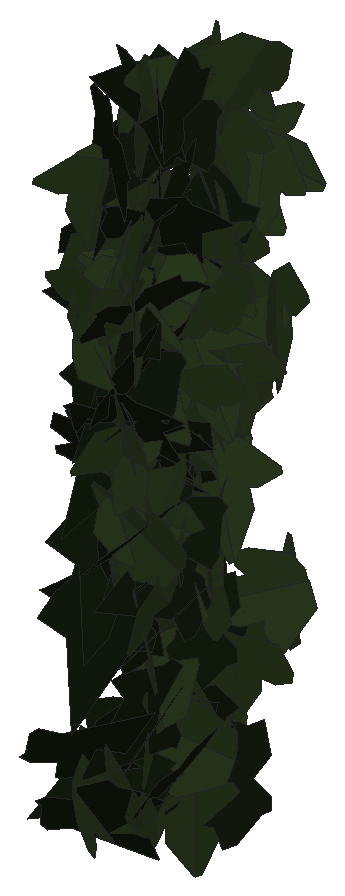
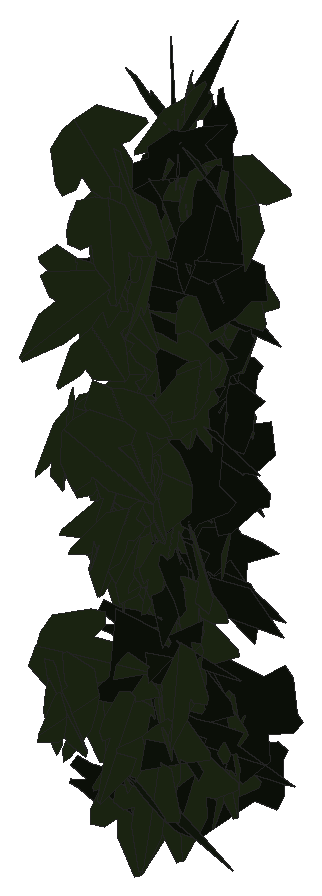
# SketchUp Ruby script. Lengths in inches.
U = 1.inch
M = Sketchup.active_model
def pt(a) = Geom::Point3d.new(a.map { |v| v * U })
def face(e, loops, mat)
  f = e.add_face(loops[0].map { |a| pt(a) })
  loops[1..].each { |l| e.add_face(l.map { |a| pt(a) }).erase! }
  f.material = f.back_material = mat if mat
  f
end
# faces: each face lists its corners as indices into pts; further lists are holes
def faces(e, pts, list, mat = nil) = list.each { |f| face(e, (f[0].is_a?(Array) ? f : [f]).map { |l| l.map { |i| pts[i] } }, mat) }
# xy, xz, yz: faces in a plane at the given z, y or x. An outline is a flat list of corners, or four numbers for a rectangle; further outlines are holes
def ring(l) = l.size == 4 ? [[l[0], l[1]], [l[2], l[1]], [l[2], l[3]], [l[0], l[3]]] : l.each_slice(2).to_a
def flat(e, list, mat, &to3) = list.each { |f| face(e, (f[0].is_a?(Array) ? f : [f]).map { |l| ring(l).map { |u, v| to3.(u, v) } }, mat) }
def xy(e, z, list, mat = nil) = flat(e, list, mat) { |x, y| [x, y, z] }
def xz(e, y, list, mat = nil) = flat(e, list, mat) { |x, z| [x, y, z] }
def yz(e, x, list, mat = nil) = flat(e, list, mat) { |y, z| [x, y, z] }
def lines(e, pts, list) = list.each { |a, b| e.add_line(pt(pts[a]), pt(pts[b])) }
# prism: a flat outline (further loops are holes) pulled along v
def prism(e, loops, v, mat = nil)
  f = face(e, loops, mat); d = Geom::Vector3d.new(v.map { |x| x * U })
  f.pushpull(f.normal.samedirection?(d) ? d.length : -d.length)
end
def box(e, o, s, mat = nil) = prism(e, [[o, [o[0] + s[0], o[1], o[2]], [o[0] + s[0], o[1] + s[1], o[2]], [o[0], o[1] + s[1], o[2]]]], [0, 0, s[2]], mat)
def at(x, y, z, deg = 0) = Geom::Transformation.translation(pt([x, y, z])) * Geom::Transformation.rotation(ORIGIN, Z_AXIS, deg.degrees)
def axes(o, x, y, z) = Geom::Transformation.new([*x, 0, *y, 0, *z, 0, *pt(o).to_a, 1])
def part(name) = M.definitions.add(name)
# library, detail: a bought-in or finely detailed component or shape, given as its bounding box
def library(name, o, s) = part(name).tap { |d| box(d.entities, o, s) }
def detail(e, o, s) = box(e.add_group.entities, o, s)
def put(e, d, t, mat = nil) = e.add_instance(d, t).tap { |i| i.material = mat if mat }
def group(e, t, mat = nil) = e.add_group.tap { |g| g.transformation = t; g.material = mat if mat }.entities
root = M.entities
M.materials.add("efeu1").color = [18, 25, 13]
M.materials.add("efeu2").color = [43, 57, 29]
c1 = part("ivyleaf_10")
p = [[0,0.5,-0.03],[-0.0625,2.02,-0.43],[-0.19,2.01,-0.46],[-0.54,1.05,-0.29],[-0.52,0.625,-0.18],[-0.83,0.76,-0.28],
  [-1.16,0.64,-0.33],[-1.15,0.33,-0.24],[-0.77,-0.39,0.02],[-0.3,-0.51,0.16],[0.04,-0.48,0.23],[-0.02,2.01,-0.4375],
  [-0.06,2.01,-0.43],[0.04,-0.49,0.23],[0.67,-0.49,0.14],[1.38,0.36,-0.2],[1.375,0.51,-0.24],[0.81,0.65,-0.19],
  [0.62,0.59,-0.15],[0.6,1.09,-0.28],[0.5,1.23,-0.31]]
faces(c1.entities,p,[[0,1,2,3,4,5,6,7,8,9,10],[11,12,0,13,14,15,16,17,18,19,20]],"efeu2")
c2 = part("ivyleaf_9")
p = [[1.54,2.16,1.25],[1.36,2.04,1.19],[-0.21,0.99,0.68],[-0.71,1.11,0.82],[-0.85,0.86,0.67],[-0.8,0.17,0.21],
  [-0.9,-0.01,0.1],[-0.67,-0.16,-0.02],[-0.08,-0.08,-0.05],[-0.03,-0.6,-0.4],[0.65,-0.88,-0.66],[0.83,-0.6,-0.49],
  [1.29,-0.42,-0.43],[1.8125,-0.07,-0.26],[1.21,0.44,0.15]]
faces(c2.entities,p,[[0,1,2,3,4,5,6,7,8,9,10,11,12,13,14]],"efeu1")
put(root,c1,axes([52.67,225.2,214.57],[-0.47031,0.14303,0.0914],[-0.086,0.03132,-0.49155],[-0.14634,-0.47808,-0.00486]))
put(root,c1,axes([52.51,224.59,219.58],[0.08051,0.49259,-0.02963],[-0.0071,-0.02886,-0.49912],[-0.49342,0.08079,0.00235]))
put(root,c2,axes([52.39,224.03,220.99],[0.04906,0.27924,-0.41185],[0.05314,0.40854,0.28332],[0.49474,-0.07157,0.01041]))
put(root,c1,axes([52.78,223.59,220.3],[-0.47435,-0.01429,0.15743],[-0.15723,-0.00901,-0.47455],[0.0164,-0.49971,0.00405]))
put(root,c1,axes([52.55,224.14,220.64],[-0.42295,-0.19138,-0.1857],[0.17438,0.06493,-0.46408],[0.20175,-0.45734,0.01182]))
put(root,c1,axes([52.6875,223.55,214.39],[-0.17216,0.35629,0.30564],[-0.14577,0.26888,-0.39555],[-0.44622,-0.2253,0.01129]))
put(root,c2,axes([52.23,223.99,218.2],[0.39606,-0.04788,0.3014],[0.30252,-0.00339,-0.39808],[0.04016,0.49769,0.02629]))
put(root,c1,axes([52.74,223.76,221.7],[-0.36486,-0.33384,0.07369],[-0.05206,-0.05227,-0.49453],[0.33789,-0.36854,0.00338]))
put(root,c1,axes([52.9,223.76,214.5625],[-0.37475,0.06828,0.32388],[-0.31854,0.05856,-0.38092],[-0.08995,-0.49184,-0.00039]))
put(root,c2,axes([52.52,224.625,221.7],[-0.03774,0.03706,-0.49719],[0.36563,-0.33693,-0.05287],[-0.33896,-0.36757,-0.00167]))
put(root,c1,axes([52.65,225.77,219.73],[0.49131,-0.03644,-0.08536],[-0.084,0.02106,-0.49244],[0.03949,0.49823,0.01457]))
put(root,c1,axes([52.55,224.3125,219.3125],[-0.06415,-0.14282,-0.47485],[0.20027,0.43056,-0.15656],[0.45362,-0.21029,0.00196]))
put(root,c1,axes([52.38,224.63,217.08],[0.13551,-0.15875,-0.45435],[0.28268,-0.35577,0.20861],[-0.38952,-0.31341,-0.00667]))
put(root,c1,axes([52.93,226.08,219.28],[0.28536,0.02931,-0.40952],[-0.41056,0.02424,-0.28435],[0.00319,0.49855,0.0379]))
put(root,c2,axes([52.36,223.57,214.65],[0.38465,0.30494,-0.09515],[0.07137,0.06313,0.49084],[0.31137,-0.39118,0.00504]))
put(root,c2,axes([52.79,224.2,218.59],[-0.47841,-0.06703,-0.12897],[0.12928,0.0065,-0.48295],[0.06643,-0.49544,0.01111]))
put(root,c1,axes([52.78,224.67,215.85],[-0.48658,0.0993,0.05815],[-0.06589,-0.03325,-0.49452],[-0.09434,-0.48891,0.04545]))
put(root,c1,axes([52.82,225.84,222.07],[-0.48769,0.04965,0.09845],[-0.10624,-0.09202,-0.47984],[-0.02953,-0.48895,0.1003]))
put(root,c2,axes([52.98,224.24,214.69],[-0.46724,-0.08366,0.15713],[-0.14927,-0.05634,-0.47386],[0.09699,-0.48972,0.02767]))
put(root,c2,axes([53.11,223.84,216.68],[-0.1279,0.05617,-0.48009],[-0.43988,-0.21938,0.09152],[-0.20036,0.44578,0.10554]))
put(root,c1,axes([52.59,224,217.57],[-0.28606,0.26784,-0.31053],[0.16021,-0.27553,-0.38524],[-0.37749,-0.31991,0.07182]))
put(root,c2,axes([52.87,224.57,217.93],[0.29894,-0.02657,0.39991],[-0.37744,0.14917,0.29205],[-0.13483,-0.47649,0.06913]))
put(root,c2,axes([53.02,224.95,214.39],[-0.44389,0.22991,-0.01027],[-0.0307,-0.08127,-0.4924],[-0.22809,-0.4365,0.08626]))
put(root,c2,axes([52.77,224.23,217.22],[-0.35232,-0.34422,-0.08592],[0.05215,0.06953,-0.49239],[0.35093,-0.35592,-0.01309]))
put(root,c1,axes([52.46,223.89,221.51],[-0.2735,0.05829,-0.41449],[0.38893,-0.14761,-0.27739],[-0.1547,-0.47415,0.0354]))
put(root,c2,axes([52.65,223.49,214.3],[0.39223,0.3092,0.02341],[0.01729,0.01589,-0.49945],[-0.30961,0.39261,0.00177]))
put(root,c1,axes([53.08,225.23,222.17],[-0.04988,0.09594,0.48817],[-0.46362,0.169,-0.08059],[-0.18046,-0.46069,0.0721]))
put(root,c1,axes([52.75,225.21,221.28],[-0.36684,0.33929,-0.0177],[0.01453,-0.01035,-0.49968],[-0.33944,-0.36712,-0.00227]))
put(root,c1,axes([52.82,224.55,214.32],[-0.28191,-0.41198,0.02827],[0.02725,-0.05271,-0.49647],[0.41205,-0.27837,0.05218]))
put(root,c2,axes([53.03,223.5625,222.35],[0.13727,-0.00209,-0.48078],[-0.48061,0.01282,-0.13728],[0.0129,0.49983,0.0015]))
put(root,c2,axes([52.6,224.23,219.23],[-0.06176,-0.16374,-0.46838],[0.11691,0.4539,-0.17409],[0.4822,-0.13102,-0.01778]))
put(root,c2,axes([52.78,223.87,216.59],[-0.40331,-0.19849,-0.21895],[0.22498,0.034,-0.44523],[0.19164,-0.45765,0.06188]))
put(root,c2,axes([52.48,224.04,219.42],[0.164,-0.29974,0.36504],[0.16506,-0.32569,-0.34158],[0.44256,0.23255,-0.00788]))
put(root,c1,axes([52.95,223.88,214.06],[-0.48423,0.01835,-0.12323],[-0.12305,0.00729,0.48457],[0.01958,0.49961,-0.00255]))
put(root,c1,axes([52.74,225.66,218.12],[0.04747,0.49323,0.0669],[0.01556,0.0657,-0.49542],[-0.4975,0.04911,-0.00912]))
put(root,c1,axes([52.57,224.14,220.5],[0.00643,-0.10196,-0.48945],[0.26962,-0.4115,0.08927],[-0.42103,-0.26508,0.04969]))
put(root,c1,axes([52.77,224.8,217.47],[-0.06383,0.48781,-0.08927],[0.01488,-0.08808,-0.49196],[-0.49569,-0.06545,-0.00327]))
put(root,c2,axes([53.24,223.76,220.34],[-0.14275,-0.04655,-0.47692],[-0.445,-0.17173,0.14996],[-0.17777,0.46727,0.0076]))
put(root,c1,axes([52.92,224.43,216.01],[-0.29253,-0.40549,-0.00238],[0.00081,0.00235,-0.49999],[0.40549,-0.29253,-0.00072]))
put(root,c1,axes([53.12,225.45,218.88],[-0.34442,-0.23695,0.27428],[-0.22149,-0.16191,-0.418],[0.28691,-0.40944,0.00656]))
put(root,c1,axes([52.85,225.11,214.93],[0.17079,0.44738,-0.14379],[-0.05001,-0.13482,-0.47888],[-0.46726,0.17796,-0.0013]))
put(root,c1,axes([53,224.77,214.94],[-0.46044,-0.18717,0.05443],[-0.04451,-0.03497,-0.49679],[0.18978,-0.46232,0.01554]))
put(root,c1,axes([53.17,224.68,217.94],[0.02867,-0.05408,-0.49624],[-0.30947,0.38808,-0.06017],[0.39167,0.31059,-0.01122]))
put(root,c2,axes([53.02,224.17,214.89],[0.07396,0.28565,0.40365],[0.01202,0.40698,-0.29021],[-0.49435,0.05264,0.05333]))
put(root,c1,axes([52.91,225.89,220.58],[0.09942,0.41365,-0.26269],[-0.07969,-0.25082,-0.42513],[-0.48349,0.1264,0.01606]))
put(root,c1,axes([53.07,224.64,217.06],[0.15443,-0.16313,0.4467],[-0.27663,0.35121,0.22389],[-0.38682,-0.31629,0.01822]))
put(root,c1,axes([53.05,225.38,218.39],[-0.14687,0.28374,0.3846],[-0.21694,0.31894,-0.31815],[-0.42587,-0.26032,0.02942]))
put(root,c1,axes([52.96,225.21,215.32],[-0.04841,-0.37045,-0.3323],[0.04369,0.32941,-0.3736],[0.49573,-0.06521,0.00048]))
put(root,c1,axes([52.85,223.52,219.86],[0.02906,0.06102,0.49541],[0.03372,0.49488,-0.06293],[-0.49801,0.03707,0.02465]))
put(root,c2,axes([52.8,224.51,216.84],[-0.04935,0.36444,0.33874],[0.02627,-0.33802,0.36749],[0.49686,0.05407,0.01422]))
put(root,c2,axes([52.98,224.05,220.58],[0.27036,0.41314,-0.07886],[-0.04953,-0.06182,-0.49369],[-0.41767,0.27476,0.00749]))
put(root,c1,axes([53.31,223.49,218.61],[0.04614,-0.0074,-0.49781],[-0.43277,0.24656,-0.04377],[0.24612,0.43492,0.01635]))
put(root,c1,axes([52.65,224.5,219.61],[0.27722,0.02992,-0.41503],[0.39918,0.12168,0.27541],[0.11748,-0.48404,0.04358]))
put(root,c1,axes([53.32,225.03,220.79],[-0.22036,0.02908,0.44788],[-0.44535,0.04772,-0.22222],[-0.05567,-0.49687,0.00487]))
put(root,c2,axes([53.35,224.83,220.6],[-0.15135,0.05969,0.47279],[-0.47648,-0.01069,-0.15118],[-0.00794,-0.49631,0.06012]))
put(root,c2,axes([52.98,224.82,215.64],[-0.24299,-0.18677,0.39506],[0.31337,0.24058,0.30647],[-0.30456,0.39654,0.00014]))
put(root,c1,axes([52.93,225.43,217.39],[-0.00889,-0.17053,-0.46994],[0.00141,-0.47002,0.17053],[-0.49992,0.00171,0.00884]))
put(root,c1,axes([53.18,224.1875,215.35],[0.38537,-0.01228,0.31834],[-0.31681,0.03785,0.38497],[-0.03355,-0.49841,0.0214]))
put(root,c1,axes([52.93,224.42,216.64],[0.49634,0.06032,0.00318],[0.00301,0.00161,-0.49999],[-0.06033,0.49634,0.00123]))
put(root,c2,axes([53.07,224.68,222.29],[-0.25567,-0.39051,0.17926],[-0.09342,-0.15308,-0.46673],[0.41941,-0.27215,0.00531]))
put(root,c1,axes([52.68,224.78,218.3125],[-0.07433,0.02926,-0.49358],[0.43572,-0.23205,-0.07938],[-0.23371,-0.44193,0.009]))
put(root,c1,axes([53.125,223.7,221.38],[0.25045,-0.39558,-0.17547],[-0.09406,0.14813,-0.4682],[0.4224,0.26753,-0.00022]))
put(root,c1,axes([52.91,224.58,215.21],[0.17161,-0.33144,0.33271],[0.20826,-0.26378,-0.37019],[0.42092,0.26564,0.04752]))
put(root,c1,axes([53.11,223.75,221.21],[0.36568,-0.31479,-0.13109],[-0.09591,0.08951,-0.48248],[0.32723,0.37802,0.00508]))
put(root,c1,axes([52.98,224.58,218.13],[0.06617,0.4189,0.26484],[0.01275,0.26566,-0.42339],[-0.49544,0.06278,0.02447]))
put(root,c1,axes([52.9,225.99,221.08],[0.10989,0.25178,0.41777],[0.1221,0.4004,-0.27344],[-0.47224,0.16212,0.02652]))
put(root,c1,axes([53.07,225.21,221.8],[-0.48743,-0.08118,-0.07632],[0.0744,0.01783,-0.49411],[0.08294,-0.49304,-0.00531]))
put(root,c2,axes([53.18,224.1875,215.23],[0.22771,0.36005,-0.26175],[-0.13471,-0.22449,-0.42598],[-0.42426,0.26452,-0.00523]))
put(root,c1,axes([53.43,226.04,215.82],[-0.05259,0.08371,0.49013],[-0.47374,0.14125,-0.07496],[-0.15101,-0.47227,0.06446]))
put(root,c1,axes([53.04,224.18,222.68],[0.05283,0.49251,-0.06815],[-0.01905,-0.06647,-0.4952],[-0.49684,0.05492,0.01174]))
put(root,c1,axes([53.0625,224.24,219.51],[-0.09401,0.48643,0.06744],[-0.02236,0.06435,-0.49534],[-0.49057,-0.09615,0.00966]))
put(root,c1,axes([53.37,224.11,220.33],[0.10997,0.22398,0.43329],[-0.32605,-0.29659,0.23606],[0.36276,-0.33447,0.08083]))
put(root,c2,axes([53.47,224.71,216.11],[-0.42743,0.06376,0.25147],[-0.25432,-0.00726,-0.43043],[-0.05124,-0.49586,0.03864]))
put(root,c2,axes([53.28,224.09,217.07],[-0.03556,0.4676,0.17345],[-0.02181,0.17226,-0.46888],[-0.49826,-0.04091,0.00814]))
put(root,c1,axes([53.08,224.26,217.99],[-0.15067,0.4746,0.04527],[-0.01123,0.04393,-0.49794],[-0.47663,-0.15107,-0.00258]))
put(root,c1,axes([52.82,223.66,220.38],[-0.23481,-0.00547,-0.4414],[0.4404,-0.03707,-0.23382],[-0.03017,-0.49859,0.02223]))
put(root,c1,axes([53.24,223.875,221.23],[0.22879,-0.37142,-0.24433],[-0.1119,0.21783,-0.43592],[0.43027,0.25415,0.01656]))
put(root,c2,axes([53.3,223.91,219.68],[-0.49266,-0.04881,-0.07005],[0.06882,0.01574,-0.49499],[0.05052,-0.49736,-0.00879]))
put(root,c1,axes([53.21,225.76,215.66],[0.0706,-0.04746,0.49271],[-0.18456,0.45928,0.07069],[-0.4593,-0.19185,0.04733]))
put(root,c2,axes([53.09,224.2,222.42],[0.28468,-0.39875,-0.09981],[0.05904,-0.08049,0.48994],[-0.40679,-0.29073,0.00126]))
put(root,c2,axes([53.32,223.49,217.67],[0.02459,0.48504,0.11888],[-0.07242,0.12123,-0.47964],[-0.49412,0.00637,0.07622]))
put(root,c1,axes([53.08,223.65,219.45],[-0.18765,0.45072,-0.10789],[0.04498,-0.09813,-0.48821],[-0.46126,-0.19293,-0.00372]))
put(root,c1,axes([53.21,223.85,222.63],[0.1491,-0.25727,-0.40197],[-0.02999,0.41525,-0.27689],[0.47631,0.10668,0.10839]))
put(root,c2,axes([53.43,223.86,221.4],[-0.11297,0.3624,0.32543],[-0.12599,0.30096,-0.37888],[-0.47049,-0.16761,0.02332]))
put(root,c2,axes([53.32,223.98,216.35],[0.05699,0.4334,0.24273],[-0.0463,0.2479,-0.43174],[-0.49458,0.02673,0.06839]))
put(root,c1,axes([53.1875,223.66,218.77],[-0.27652,-0.3946,-0.13352],[0.07773,0.10856,-0.48184],[0.40926,-0.28723,0.00131]))
put(root,c1,axes([53.55,224.62,216.68],[-0.15949,0.11312,0.46018],[-0.46877,0.03348,-0.1707],[-0.06944,-0.48588,0.09538]))
put(root,c2,axes([53.38,224.3,215.49],[0.008,0.12122,-0.48502],[-0.07965,-0.47857,-0.12093],[-0.49355,0.0792,0.01165]))
put(root,c1,axes([53.18,224.42,215.54],[-0.46023,0.18577,-0.0606],[0.05467,-0.02645,-0.4963],[-0.18761,-0.46345,0.00404]))
put(root,c1,axes([53.07,223.67,220.49],[-0.15043,-0.22026,-0.42291],[0.252,0.33975,-0.26658],[0.4048,-0.29335,0.0088]))
put(root,c2,axes([53.05,223.4,219.13],[0.45657,0.20332,0.01439],[0.01141,0.00974,-0.49977],[-0.20351,0.45669,0.00425]))
put(root,c2,axes([53.29,223.6,220.4],[0.13497,0.48075,-0.02577],[-0.01812,-0.02167,-0.4992],[-0.4811,0.13569,0.01157]))
put(root,c1,axes([53.11,223.78,219.96],[0.04303,-0.20608,0.45352],[0.03931,0.45519,0.20311],[-0.49659,0.01818,0.05538]))
put(root,c2,axes([53.21,223.62,218.94],[0.36703,0.3051,-0.149],[-0.11339,-0.09668,-0.47728],[-0.32005,0.38415,-0.00178]))
put(root,c1,axes([53.27,224.55,219.04],[-0.364,-0.34146,-0.03012],[0.02232,0.02024,-0.49909],[0.34206,-0.36469,0.00051]))
put(root,c1,axes([53.37,224.09,218.4],[0.34396,-0.25835,-0.25485],[-0.20472,0.15178,-0.43018],[0.29963,0.40027,-0.00137]))
put(root,c1,axes([52.94,224.09,216.53],[0.18319,-0.24617,0.39477],[0.38303,-0.16101,-0.27814],[0.26407,0.40432,0.12959]))
put(root,c1,axes([53.35,224.73,220.28],[-0.34362,-0.34632,0.10948],[-0.07376,-0.08103,-0.48785],[0.35565,-0.35142,0.00459]))
put(root,c1,axes([53.3,224.62,214.04],[-0.33993,-0.36667,0.00028],[0.00333,-0.00347,-0.49998],[0.36666,-0.33991,0.0048]))
put(root,c2,axes([53.57,224.01,222.55],[-0.32092,0.33058,0.19423],[-0.14234,0.13247,-0.46064],[-0.35602,-0.35095,0.00909]))
put(root,c1,axes([53.57,223.68,217.47],[-0.30477,0.06506,-0.391],[-0.38896,0.04585,0.31082],[0.07629,0.49363,0.02266]))
put(root,c2,axes([53.32,224.51,216.85],[-0.18326,-0.22004,0.40988],[-0.17281,-0.37681,-0.27956],[0.43192,-0.24413,0.06205]))
put(root,c2,axes([53.61,225.08,214.21],[-0.44587,0.04728,0.22129],[-0.22234,-0.00073,-0.44784],[-0.04202,-0.49776,0.02168]))
put(root,c1,axes([53.3,223.85,221.21],[-0.00869,-0.18681,-0.46371],[0.01507,0.46347,-0.18699],[0.4997,-0.01723,-0.00243]))
put(root,c2,axes([53.41,224.34,217.8],[-0.45653,-0.2039,0.00174],[-0.00144,-0.00105,-0.5],[0.20391,-0.45653,0.00037]))
put(root,c1,axes([53.25,226.07,219.42],[-0.14798,0.46856,-0.09251],[-0.03548,-0.10737,-0.48704],[-0.47628,-0.13758,0.06503]))
put(root,c1,axes([53.23,223.88,219.18],[0.49872,0,-0.03579],[-0.03579,0.00181,-0.49871],[0.00013,0.5,0.00181]))
put(root,c1,axes([53.28,224.25,217.51],[0.38424,-0.3186,-0.02923],[-0.02192,0.01936,-0.49914],[0.31918,0.38487,0.00091]))
put(root,c2,axes([53.32,223.32,219.625],[-0.13526,0.32693,-0.3533],[-0.17098,0.31041,0.35271],[0.44996,0.21624,0.02782]))
put(root,c1,axes([53.19,223.8,220.49],[-0.14791,0.38624,-0.28096],[0.07157,-0.27288,-0.41281],[-0.47223,-0.16234,0.02544]))
put(root,c1,axes([53.52,224.57,220.28],[-0.27102,-0.25654,0.33277],[-0.2024,-0.26731,-0.37092],[0.36821,-0.33576,0.04104]))
put(root,c1,axes([53.54,224.58,217.23],[-0.08374,0.21349,0.44431],[-0.3512,0.2904,-0.20573],[-0.3459,-0.34654,0.10132]))
put(root,c1,axes([53.6,225.7,216.22],[0.1399,0.06486,-0.47563],[-0.43681,-0.18825,-0.15415],[-0.19907,0.45864,0.00399]))
put(root,c1,axes([53.34,225.09,219.07],[-0.37031,-0.32814,-0.07207],[0.05391,0.04782,-0.49478],[0.33161,-0.37422,-0.00004]))
put(root,c1,axes([53.69,224.37,214.89],[-0.12586,-0.01715,-0.4836],[-0.48311,-0.02406,0.12659],[-0.02761,0.49913,-0.01052]))
put(root,c2,axes([53.14,224.17,222.01],[-0.02709,0.10465,0.48817],[0.06531,-0.48395,0.10737],[0.49498,0.06958,0.01255]))
put(root,c1,axes([53.23,225.76,221.23],[0.49658,-0.00648,0.058],[0.05802,0.00103,-0.49662],[0.00631,0.49996,0.00178]))
put(root,c2,axes([53.5,224.09,214.72],[-0.05129,0.4937,0.06029],[0.00412,0.06103,-0.49624],[-0.49735,-0.05041,-0.01032]))
put(root,c1,axes([53.48,225.12,215.6875],[-0.45222,-0.19696,0.08187],[-0.08113,-0.01868,-0.49302],[0.19727,-0.45919,-0.01507]))
put(root,c1,axes([53.25,224.76,219.26],[0.1363,0.45971,0.14175],[0.03822,0.13651,-0.47948],[-0.47954,0.14154,0.00208]))
put(root,c2,axes([53.33,223.77,221.43],[0.3675,0.33203,-0.06856],[-0.05519,-0.04117,-0.49524],[-0.33451,0.37157,0.00639]))
put(root,c1,axes([53.42,224.79,220.67],[-0.31283,-0.38808,-0.03915],[0.02682,0.02866,-0.49846],[0.38912,-0.31397,0.00289]))
put(root,c1,axes([53.27,225.01,217.81],[0.18359,0.46168,0.05613],[0.02027,0.05234,-0.49684],[-0.46463,0.18471,0.0005]))
put(root,c1,axes([53.5,225.35,222.67],[-0.18599,-0.40084,0.23395],[-0.09106,-0.21562,-0.44183],[0.4551,-0.20696,0.00721]))
put(root,c1,axes([53.14,223.67,217.9],[0.18055,0.15213,0.44075],[0.20314,0.39976,-0.2212],[-0.41969,0.25894,0.08255]))
put(root,c1,axes([53.41,223.85,216.92],[-0.00103,-0.36817,-0.3383],[0.01682,0.33808,-0.36799],[0.49972,-0.01213,0.01169]))
